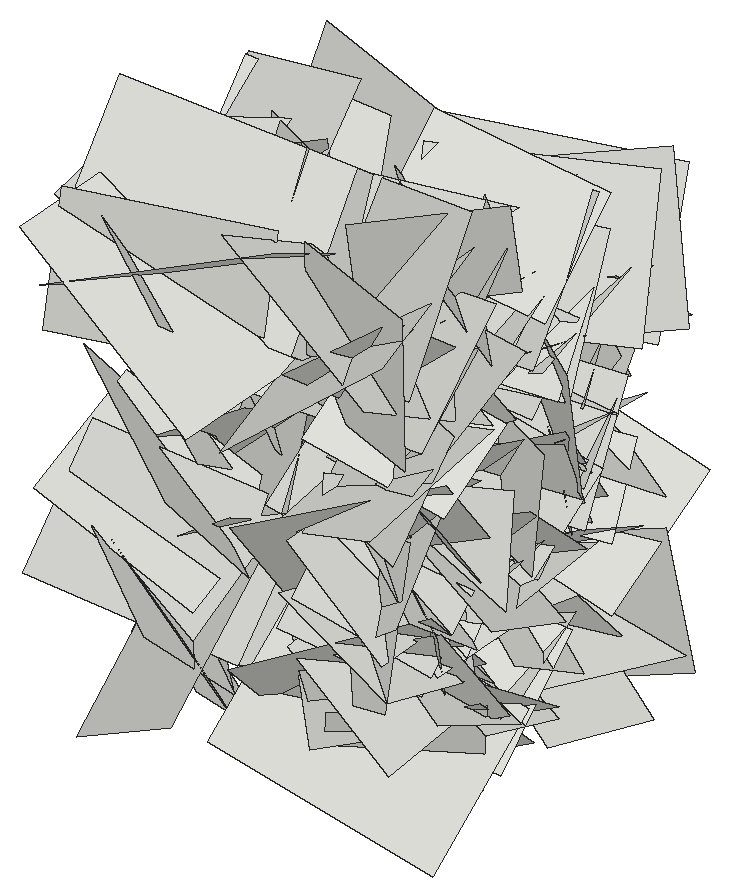
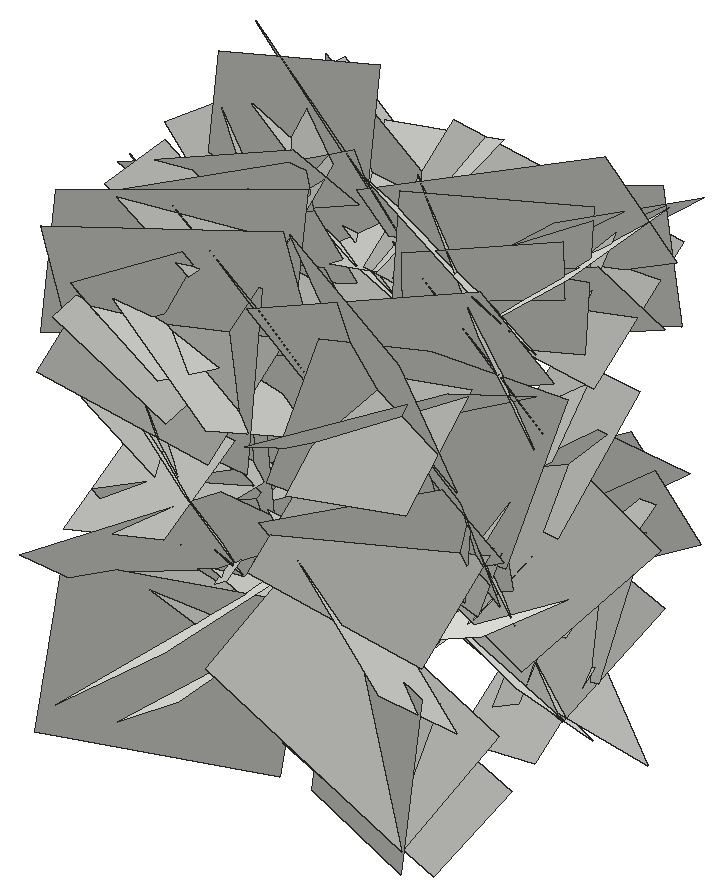
# SketchUp Ruby script. Lengths in inches.
U = 1.inch
M = Sketchup.active_model
def pt(a) = Geom::Point3d.new(a.map { |v| v * U })
def face(e, loops, mat)
  f = e.add_face(loops[0].map { |a| pt(a) })
  loops[1..].each { |l| e.add_face(l.map { |a| pt(a) }).erase! }
  f.material = f.back_material = mat if mat
  f
end
# faces: each face lists its corners as indices into pts; further lists are holes
def faces(e, pts, list, mat = nil) = list.each { |f| face(e, (f[0].is_a?(Array) ? f : [f]).map { |l| l.map { |i| pts[i] } }, mat) }
# xy, xz, yz: faces in a plane at the given z, y or x. An outline is a flat list of corners, or four numbers for a rectangle; further outlines are holes
def ring(l) = l.size == 4 ? [[l[0], l[1]], [l[2], l[1]], [l[2], l[3]], [l[0], l[3]]] : l.each_slice(2).to_a
def flat(e, list, mat, &to3) = list.each { |f| face(e, (f[0].is_a?(Array) ? f : [f]).map { |l| ring(l).map { |u, v| to3.(u, v) } }, mat) }
def xy(e, z, list, mat = nil) = flat(e, list, mat) { |x, y| [x, y, z] }
def xz(e, y, list, mat = nil) = flat(e, list, mat) { |x, z| [x, y, z] }
def yz(e, x, list, mat = nil) = flat(e, list, mat) { |y, z| [x, y, z] }
def lines(e, pts, list) = list.each { |a, b| e.add_line(pt(pts[a]), pt(pts[b])) }
# prism: a flat outline (further loops are holes) pulled along v
def prism(e, loops, v, mat = nil)
  f = face(e, loops, mat); d = Geom::Vector3d.new(v.map { |x| x * U })
  f.pushpull(f.normal.samedirection?(d) ? d.length : -d.length)
end
def box(e, o, s, mat = nil) = prism(e, [[o, [o[0] + s[0], o[1], o[2]], [o[0] + s[0], o[1] + s[1], o[2]], [o[0], o[1] + s[1], o[2]]]], [0, 0, s[2]], mat)
def at(x, y, z, deg = 0) = Geom::Transformation.translation(pt([x, y, z])) * Geom::Transformation.rotation(ORIGIN, Z_AXIS, deg.degrees)
def axes(o, x, y, z) = Geom::Transformation.new([*x, 0, *y, 0, *z, 0, *pt(o).to_a, 1])
def part(name) = M.definitions.add(name)
# library, detail: a bought-in or finely detailed component or shape, given as its bounding box
def library(name, o, s) = part(name).tap { |d| box(d.entities, o, s) }
def detail(e, o, s) = box(e.add_group.entities, o, s)
def put(e, d, t, mat = nil) = e.add_instance(d, t).tap { |i| i.material = mat if mat }
def group(e, t, mat = nil) = e.add_group.tap { |g| g.transformation = t; g.material = mat if mat }.entities
root = M.entities
c1 = part("Component\#6")
p = [[0.01,0,0],[0,3.24,4.54],[4.32,3.24,4.54],[4.33,0,0]]
faces(c1.entities,p,[[0,1,2,3]])
put(root,c1,axes([18.5,168.24,29.62],[0.00844,-0.1319,-0.59476],[0.00779,-0.59475,0.132],[-0.64572,-0.0089,-0.00618]))
put(root,c1,axes([14.53,168.37,37.02],[-0.06582,-0.55881,-0.84289],[0.17414,-0.83883,0.54402],[1.05774,0.10333,-0.14201]))
put(root,c1,axes([14.53,162.55,24.47],[0.08094,0.6993,-0.63815],[0.06519,-0.64254,-0.69674],[1.00139,-0.01469,0.09694]))
put(root,c1,axes([18.5,167.47,38.84],[0.19203,-0.25676,-0.78485],[0.09527,-0.79261,0.28005],[-0.87013,-0.14344,-0.14255]))
put(root,c1,axes([18.5,168.14,25.37],[0.00005,-0.54267,0.44601],[0.16088,0.43548,0.52984],[-0.72699,0.09633,0.11728]))
put(root,c1,axes([14.53,169.13,31.47],[0.22896,-0.22184,-0.76377],[0.12794,-0.77313,0.25869],[0.83329,0.17965,0.17014]))
put(root,c1,axes([14.53,164.67,22.86],[-0.07455,-1.03669,0.46758],[0.01691,0.46753,1.03897],[1.20537,-0.07068,0.01434]))
put(root,c1,axes([18.5,161.42,33.85],[0.12931,-0.58697,0.4315],[0.06321,0.44408,0.58723],[-0.76963,-0.06214,0.12073]))
put(root,c1,axes([14.53,160.7,27.63],[-0.09928,0.64406,-0.88513],[0.13228,-0.87629,-0.65083],[1.15276,0.15602,-0.00154]))
put(root,c1,axes([14.53,159.57,38.3125],[-0.19748,1.37219,0.09956],[-0.15298,0.08042,-1.37849],[1.4503,0.19533,-0.13185]))
put(root,c1,axes([18.5,165.91,24.52],[-0.03596,-0.58924,0.24858],[0.15481,0.23521,0.57749],[-0.65999,0.08727,0.12191]))
put(root,c1,axes([14.53,166.55,31.56],[0.0814,0.41102,-0.8284],[0.17089,-0.82447,-0.39413],[0.96524,0.11131,0.13964]))
put(root,c1,axes([18.5,169.1,21.1],[0.05323,-0.42134,0.48328],[0.06346,0.48572,0.41725],[-0.67666,0.01241,0.07715]))
put(root,c1,axes([14.53,166.67,25.47],[-0.29316,-1.18227,0.54308],[0.10516,0.53443,1.21398],[1.37509,-0.29293,0.02294]))
put(root,c1,axes([14.53,168.75,37.98],[-0.06882,-0.53698,-1.12739],[-0.1022,-1.12338,0.54063],[1.31971,-0.115,-0.01692]))
put(root,c1,axes([14.53,158.58,28.72],[0.17742,0.80309,0.64454],[-0.10421,0.66248,-0.79991],[1.08655,-0.0676,-0.18196]))
put(root,c1,axes([18.5,163.1,21.29],[0.03251,-0.459,0.52355],[0.17075,0.51451,0.44164],[-0.71801,0.10157,0.12873]))
put(root,c1,axes([14.53,169.04,36.23],[-0.04162,0.78981,-0.64322],[0.24351,-0.62024,-0.77563],[1.05189,0.17484,0.15411]))
put(root,c1,axes([14.53,170.89,20.28],[0.12274,-1.02279,0.17958],[-0.0333,0.17716,1.02926],[1.10024,0.11946,0.01112]))
put(root,c1,axes([14.53,167.53,29.6],[0.04916,0.6172,0.8297],[0.08211,0.82613,-0.61887],[1.09305,-0.08981,0.00917]))
put(root,c1,axes([14.53,171.44,27.64],[0.05126,-0.8571,0.56567],[0.11133,0.56746,0.85083],[1.08285,-0.01777,-0.11425]))
put(root,c1,axes([18.5,163.13,28.77],[0.13219,-0.55975,0.33448],[0.05965,0.34851,0.56225],[-0.68862,-0.07726,0.11291]))
put(root,c1,axes([14.53,163.625,35.04],[0.27654,-0.44632,0.88094],[-0.09901,0.89592,0.48157],[1.04211,0.20356,-0.18801]))
put(root,c1,axes([14.53,167.41,29.34],[-0.20833,-0.42173,1.22713],[0.0869,1.23461,0.43743],[1.37269,-0.14217,0.15855]))
put(root,c1,axes([14.53,168.84,39.14],[0.0295,-0.69575,-0.73723],[0.22295,-0.71749,0.68506],[1.05113,0.17171,-0.12461]))
put(root,c1,axes([14.53,163.85,26.9],[0.03329,1.04875,0.11229],[0.24045,0.10299,-1.02538],[1.09187,-0.05466,0.22238]))
put(root,c1,axes([14.53,160.22,28.4],[0.15479,0.80897,-0.76348],[-0.02106,-0.76802,-0.81757],[1.17891,-0.11994,0.08565]))
put(root,c1,axes([14.53,169.63,32.59],[0.01533,-0.4611,-1.03377],[0.17767,-1.02158,0.45801],[1.18663,0.15892,-0.05522]))
put(root,c1,axes([14.53,159.8,34.2],[-0.03301,0.77795,0.85676],[0.24326,0.8442,-0.75821],[1.20233,-0.14944,0.17692]))
put(root,c1,axes([14.53,166.97,25.06],[-0.03339,-0.82276,-0.77538],[0.30966,-0.75526,0.78954],[1.15769,0.17829,-0.23355]))
put(root,c1,axes([14.53,165.55,34.43],[-0.04885,1.13911,0.54464],[0.08516,0.54654,-1.13629],[1.33566,0.00681,0.09237]))
put(root,c1,axes([14.53,164.92,23.28],[0.02573,-1.02703,-0.88101],[-0.12942,-0.87922,1.02158],[1.42847,-0.06116,0.10843]))
put(root,c1,axes([14.53,160.96,32.62],[0.12215,0.75895,-0.88724],[0.014,-0.89234,-0.7616],[1.23753,-0.06482,0.09619]))
put(root,c1,axes([14.53,172.54,38.57],[-0.12011,-0.4932,-1.18141],[0.20578,-1.17893,0.47355],[1.34134,0.1367,-0.17844]))
put(root,c1,axes([14.53,171.44,26.6],[-0.03428,0.27698,-1.26013],[0.06702,-1.25867,-0.27828],[1.36598,0.0687,-0.01797]))
put(root,c1,axes([14.53,173.53,27.66],[0.08068,-0.97468,-0.75893],[0.01331,-0.75972,0.97695],[1.30935,0.06778,0.03684]))
put(root,c1,axes([14.53,158.99,33.95],[0.09747,0.08794,1.12692],[0.17247,1.11783,-0.1005],[1.18568,-0.16983,-0.07802]))
put(root,c1,axes([14.53,166.62,31.96],[0.21061,0.75098,-0.921],[-0.02022,-0.93165,-0.76377],[1.25951,-0.14053,0.14175]))
put(root,c1,axes([14.53,158.06,26.05],[0.19995,0.52409,1.06255],[0.00833,1.07535,-0.5318],[1.25583,-0.09057,-0.16565]))
put(root,c1,axes([14.53,172.42,21.79],[0.22827,-1.35966,0.24048],[-0.1567,0.21929,1.3722],[1.45519,0.2369,0.11004]))
put(root,c1,axes([14.53,165.11,34.6875],[0.03998,0.77126,1.05992],[0.2457,1.03973,-0.76482],[1.36759,-0.20934,0.10642]))
put(root,c1,axes([14.53,159.18,36.25],[0.04304,0.74935,1.15311],[0.14712,1.14549,-0.74928],[1.45028,-0.13844,0.04179]))
put(root,c1,axes([14.53,168.45,29.92],[0.2904,-0.81126,-1.09363],[-0.15157,-1.12651,0.79984],[1.4354,0.04517,0.30571]))
put(root,c1,axes([14.53,157.9,37.93],[0.24747,1.3445,0.30187],[-0.11522,0.32319,-1.35538],[1.4561,-0.20293,-0.15855]))
put(root,c1,axes([14.53,163.2,33.68],[0.16473,-1.2102,0.57798],[0.2383,0.59712,1.18983],[1.40149,0.04071,-0.27024]))
put(root,c1,axes([28.31,163.2,33.68],[-0.16473,-1.2102,0.57798],[-0.2383,0.59712,1.18983],[-1.40149,0.04071,-0.27024]))
put(root,c1,axes([28.31,157.9,37.93],[-0.24747,1.3445,0.30187],[0.11522,0.32319,-1.35538],[-1.4561,-0.20293,-0.15855]))
put(root,c1,axes([28.31,168.45,29.92],[-0.2904,-0.81126,-1.09363],[0.15157,-1.12651,0.79984],[-1.4354,0.04517,0.30571]))
put(root,c1,axes([28.31,159.18,36.25],[-0.04304,0.74935,1.15311],[-0.14712,1.14549,-0.74928],[-1.45028,-0.13844,0.04179]))
put(root,c1,axes([28.31,165.11,34.6875],[-0.03998,0.77126,1.05992],[-0.2457,1.03973,-0.76482],[-1.36759,-0.20934,0.10642]))
put(root,c1,axes([28.31,172.42,21.79],[-0.22827,-1.35966,0.24048],[0.1567,0.21929,1.3722],[-1.45519,0.2369,0.11004]))
put(root,c1,axes([28.31,158.06,26.05],[-0.19995,0.52409,1.06255],[-0.00833,1.07535,-0.5318],[-1.25583,-0.09057,-0.16565]))
put(root,c1,axes([28.31,166.62,31.96],[-0.21061,0.75098,-0.921],[0.02022,-0.93165,-0.76377],[-1.25951,-0.14053,0.14175]))
put(root,c1,axes([28.31,158.99,33.95],[-0.09747,0.08794,1.12692],[-0.17247,1.11783,-0.1005],[-1.18568,-0.16983,-0.07802]))
put(root,c1,axes([28.31,173.53,27.66],[-0.08068,-0.97468,-0.75893],[-0.01331,-0.75972,0.97695],[-1.30935,0.06778,0.03684]))
put(root,c1,axes([28.31,171.44,26.6],[0.03428,0.27698,-1.26013],[-0.06702,-1.25867,-0.27828],[-1.36598,0.0687,-0.01797]))
put(root,c1,axes([28.31,172.54,38.57],[0.12011,-0.4932,-1.18141],[-0.20578,-1.17893,0.47355],[-1.34134,0.1367,-0.17844]))
put(root,c1,axes([28.31,160.96,32.62],[-0.12215,0.75895,-0.88724],[-0.014,-0.89234,-0.7616],[-1.23753,-0.06482,0.09619]))
put(root,c1,axes([28.31,164.92,23.28],[-0.02573,-1.02703,-0.88101],[0.12942,-0.87922,1.02158],[-1.42847,-0.06116,0.10843]))
put(root,c1,axes([28.31,165.55,34.43],[0.04885,1.13911,0.54464],[-0.08516,0.54654,-1.13629],[-1.33566,0.00681,0.09237]))
put(root,c1,axes([28.31,166.97,25.06],[0.03339,-0.82276,-0.77538],[-0.30966,-0.75526,0.78954],[-1.15769,0.17829,-0.23355]))
put(root,c1,axes([28.31,159.8,34.2],[0.03301,0.77795,0.85676],[-0.24326,0.8442,-0.75821],[-1.20233,-0.14944,0.17692]))
put(root,c1,axes([28.31,169.63,32.59],[-0.01533,-0.4611,-1.03377],[-0.17767,-1.02158,0.45801],[-1.18663,0.15892,-0.05522]))
put(root,c1,axes([28.31,160.22,28.4],[-0.15479,0.80897,-0.76348],[0.02106,-0.76802,-0.81757],[-1.17891,-0.11994,0.08565]))
put(root,c1,axes([28.31,163.85,26.9],[-0.03329,1.04875,0.11229],[-0.24045,0.10299,-1.02538],[-1.09187,-0.05466,0.22238]))
put(root,c1,axes([28.31,168.84,39.14],[-0.0295,-0.69575,-0.73723],[-0.22295,-0.71749,0.68506],[-1.05113,0.17171,-0.12461]))
put(root,c1,axes([28.31,167.41,29.34],[0.20833,-0.42173,1.22713],[-0.0869,1.23461,0.43743],[-1.37269,-0.14217,0.15855]))
put(root,c1,axes([28.31,163.625,35.04],[-0.27654,-0.44632,0.88094],[0.09901,0.89592,0.48157],[-1.04211,0.20356,-0.18801]))
put(root,c1,axes([24.34,163.13,28.77],[-0.13219,-0.55975,0.33448],[-0.05965,0.34851,0.56225],[0.68862,-0.07726,0.11291]))
put(root,c1,axes([28.31,171.44,27.64],[-0.05126,-0.8571,0.56567],[-0.11133,0.56746,0.85083],[-1.08285,-0.01777,-0.11425]))
put(root,c1,axes([28.31,167.53,29.6],[-0.04916,0.6172,0.8297],[-0.08211,0.82613,-0.61887],[-1.09305,-0.08981,0.00917]))
put(root,c1,axes([28.31,170.89,20.28],[-0.12274,-1.02279,0.17958],[0.0333,0.17716,1.02926],[-1.10024,0.11946,0.01112]))
put(root,c1,axes([28.31,169.04,36.23],[0.04162,0.78981,-0.64322],[-0.24351,-0.62024,-0.77563],[-1.05189,0.17484,0.15411]))
put(root,c1,axes([24.34,163.1,21.29],[-0.03251,-0.459,0.52355],[-0.17075,0.51451,0.44164],[0.71801,0.10157,0.12873]))
put(root,c1,axes([28.31,158.58,28.72],[-0.17742,0.80309,0.64454],[0.10421,0.66248,-0.79991],[-1.08655,-0.0676,-0.18196]))
put(root,c1,axes([28.31,168.75,37.98],[0.06882,-0.53698,-1.12739],[0.1022,-1.12338,0.54063],[-1.31971,-0.115,-0.01692]))
put(root,c1,axes([28.31,166.67,25.47],[0.29316,-1.18227,0.54308],[-0.10516,0.53443,1.21398],[-1.37509,-0.29293,0.02294]))
put(root,c1,axes([24.34,169.1,21.1],[-0.05323,-0.42134,0.48328],[-0.06346,0.48572,0.41725],[0.67666,0.01241,0.07715]))
put(root,c1,axes([28.31,166.55,31.56],[-0.0814,0.41102,-0.8284],[-0.17089,-0.82447,-0.39413],[-0.96524,0.11131,0.13964]))
put(root,c1,axes([24.34,165.91,24.52],[0.03596,-0.58924,0.24858],[-0.15481,0.23521,0.57749],[0.65999,0.08727,0.12191]))
put(root,c1,axes([28.31,159.57,38.3125],[0.19748,1.37219,0.09956],[0.15298,0.08042,-1.37849],[-1.4503,0.19533,-0.13185]))
put(root,c1,axes([28.31,160.7,27.63],[0.09928,0.64406,-0.88513],[-0.13228,-0.87629,-0.65083],[-1.15276,0.15602,-0.00154]))
put(root,c1,axes([24.34,161.42,33.85],[-0.12931,-0.58697,0.4315],[-0.06321,0.44408,0.58723],[0.76963,-0.06214,0.12073]))
put(root,c1,axes([28.31,164.67,22.86],[0.07455,-1.03669,0.46758],[-0.01691,0.46753,1.03897],[-1.20537,-0.07068,0.01434]))
put(root,c1,axes([28.31,169.13,31.47],[-0.22896,-0.22184,-0.76377],[-0.12794,-0.77313,0.25869],[-0.83329,0.17965,0.17014]))
put(root,c1,axes([24.34,168.14,25.37],[-0.00005,-0.54267,0.44601],[-0.16088,0.43548,0.52984],[0.72699,0.09633,0.11728]))
put(root,c1,axes([24.34,167.47,38.84],[-0.19203,-0.25676,-0.78485],[-0.09527,-0.79261,0.28005],[0.87013,-0.14344,-0.14255]))
put(root,c1,axes([28.31,162.55,24.47],[-0.08094,0.6993,-0.63815],[-0.06519,-0.64254,-0.69674],[-1.00139,-0.01469,0.09694]))
put(root,c1,axes([28.31,168.37,37.02],[0.06582,-0.55881,-0.84289],[-0.17414,-0.83883,0.54402],[-1.05774,0.10333,-0.14201]))
put(root,c1,axes([24.34,168.24,29.62],[-0.00844,-0.1319,-0.59476],[-0.00779,-0.59475,0.132],[0.64572,-0.0089,-0.00618]))
put(root,c1,axes([24.34,163.79,31.02],[-0.0186,-0.39942,0.51021],[-0.04828,0.50989,0.39761],[0.68514,0.02509,0.04187]))
put(root,c1,axes([24.34,167.3,30.05],[-0.09755,-0.36279,0.79394],[-0.2327,0.7823,0.33203],[0.89554,0.16375,0.17276]))
put(root,c1,axes([24.34,166.74,28.03],[-0.20581,0.5378,0.53941],[0.0447,0.5634,-0.54654],[0.80617,0.10606,0.16802]))
put(root,c1,axes([24.34,165.16,26.22],[0.00662,-0.41647,0.48084],[-0.04981,0.47925,0.41571],[0.67246,0.0396,0.02606]))
put(root,c1,axes([28.31,162.15,25.43],[0.09766,0.84172,-0.54191],[-0.18116,-0.52299,-0.84139],[-1.04557,0.16923,0.09516]))
put(root,c1,axes([24.34,170.38,37.22],[-0.01844,-0.65259,0.06973],[-0.0154,0.07012,0.65262],[0.69551,-0.01575,0.0163]))
put(root,c1,axes([28.31,159.15,32.85],[0.28722,0.93511,0.86971],[0.00467,0.88838,-0.95656],[-1.35365,0.20148,0.18123]))
put(root,c1,axes([24.34,158.35,30.49],[-0.08461,0.81055,-0.03501],[-0.12527,-0.04642,-0.80528],[0.85081,0.07377,-0.12204]))
put(root,c1,axes([24.34,168.23,31.98],[-0.11552,-0.73847,0.10601],[0.00435,0.10653,0.74638],[0.79079,-0.10846,0.01138]))
put(root,c1,axes([24.34,162.33,29.83],[-0.22776,0.38392,-0.75072],[0.01782,-0.77261,-0.39993],[0.89361,0.11326,-0.18337]))
put(root,c1,axes([28.31,165.04,27.71],[0.04822,0.07219,0.94774],[-0.14201,0.93984,-0.06516],[-0.99746,-0.13032,0.05509]))
put(root,c1,axes([24.34,171.91,32.4],[0.07209,-0.36069,-0.54144],[-0.07785,-0.54516,0.35394],[0.6852,-0.024,0.09718]))
put(root,c1,axes([28.31,167.29,35.58],[-0.17595,-0.29467,-0.74084],[-0.05215,-0.7515,0.30993],[-0.84352,0.10793,0.13537]))
put(root,c1,axes([28.31,157.3125,32.29],[0.25179,1.05256,0.51222],[-0.06429,0.53303,-1.06718],[-1.23914,0.18623,0.15945]))
put(root,c1,axes([24.34,168.82,35.84],[0.04533,0.37689,0.51175],[-0.01637,0.51337,-0.3768],[0.67349,-0.01289,-0.04361]))
put(root,c1,axes([24.34,159.46,22.85],[-0.09982,-0.0635,0.89488],[-0.1784,0.88507,0.04509],[0.93408,0.16225,0.10424]))
put(root,c1,axes([24.34,160.06,22.6],[-0.02839,-0.24478,0.77995],[-0.15528,0.76918,0.23637],[0.85248,0.13195,0.06903]))
put(root,c1,axes([24.34,159.67,28.14],[-0.12868,0.67272,0.52517],[-0.08613,0.51893,-0.68352],[0.90053,0.14576,0.00967]))
put(root,c1,axes([24.34,158.39,26.84],[-0.02686,0.84806,0.10272],[-0.17857,0.09579,-0.83237],[0.88773,0.04493,-0.16432]))
put(root,c1,axes([24.34,169.17,27.35],[0.00515,-0.4485,-0.48712],[0.04455,-0.48594,0.44784],[0.70046,0.0342,-0.02491]))
put(root,c1,axes([28.31,161.79,25.53],[-0.01152,-0.82607,0.19056],[-0.15176,0.18963,0.81386],[-0.88572,-0.02175,-0.14193]))
put(root,c1,axes([28.31,164.2,31.01],[0.06613,-0.18181,-0.96198],[-0.02897,-0.96387,0.1804],[-1.03734,0.01533,-0.06637]))
put(root,c1,axes([24.34,169.92,30.86],[0.08798,0.07784,-0.70174],[-0.08853,-0.70052,-0.08758],[0.74315,-0.09267,0.07264]))
put(root,c1,axes([28.31,162.32,28.44],[-0.12821,-0.42216,-0.69512],[0.01339,-0.70366,0.42514],[-0.86197,0.05186,0.11]))
put(root,c1,axes([28.31,166.33,22.3],[0.05809,-0.87115,0.26873],[-0.09257,0.26296,0.87026],[-0.96191,-0.07791,-0.06752]))
put(root,c1,axes([28.31,171.77,39.47],[0.25632,-0.1505,-1.28885],[0.2021,-1.29268,0.18672],[-1.36053,-0.22038,-0.21508]))
put(root,c1,axes([24.34,167.69,34.89],[0.01272,-0.59445,-0.3878],[0.01652,-0.38754,0.59453],[0.75216,0.01856,-0.0065]))
put(root,c1,axes([24.34,168.18,25.35],[0.0356,-0.79141,-0.13903],[-0.13499,-0.14264,0.78117],[0.84098,0.01061,0.13127]))
put(root,c1,axes([28.31,163.85,33.45],[0.03445,-0.73428,-0.4148],[-0.17499,-0.41262,0.71747],[-0.87664,0.05351,-0.15952]))
put(root,c1,axes([28.31,158.45,30.92],[0.16236,0.46297,0.88251],[-0.09478,0.89566,-0.45434],[-1.05211,-0.00924,0.17712]))
put(root,c1,axes([28.31,166.53,31.68],[0.02185,0.89564,-0.0065],[-0.05171,-0.00537,-0.89456],[-0.948,0.02094,0.04865]))
put(root,c1,axes([28.31,171.21,38.93],[0.24063,-0.51313,-1.11059],[0.16085,-1.10901,0.54342],[-1.28679,-0.23458,-0.13976]))
put(root,c1,axes([24.34,171.89,34.33],[-0.10287,-0.74562,-0.1631],[0.15609,-0.17961,0.73351],[0.79385,-0.06131,-0.16536]))
put(root,c1,axes([28.31,162.43,26.35],[-0.02315,-0.70596,0.51236],[0.01203,0.51225,0.70629],[-0.92456,0.02434,-0.00364]))
put(root,c1,axes([28.31,162.61,28.57],[0.04222,-0.49534,0.62953],[-0.20196,0.60636,0.48917],[-0.82474,-0.17384,-0.08755]))
put(root,c1,axes([28.31,162.92,24.26],[-0.16568,0.16434,-0.80239],[0.1251,-0.80382,-0.18763],[-0.85913,-0.14874,0.12742]))
put(root,c1,axes([28.31,164.5,23.79],[-0.04443,0.667,0.37408],[-0.11412,0.36576,-0.66423],[-0.80255,-0.08894,0.07374]))
put(root,c1,axes([28.31,168.875,35.8],[-0.07444,0.7996,-0.0855],[-0.00091,-0.0859,-0.80263],[-0.85241,-0.06974,0.00832]))
put(root,c1,axes([24.34,164.96,33.58],[0.03363,-0.67551,-0.53197],[-0.14584,-0.52946,0.66412],[0.89967,-0.06058,0.12754]))
put(root,c1,axes([24.34,169.82,24.93],[0.00586,-0.68753,0.27068],[0.05817,0.27032,0.6855],[0.78107,-0.01497,-0.05308]))
put(root,c1,axes([28.31,164.8,26.41],[-0.06555,-0.88967,-0.10275],[0.1194,-0.1099,0.88381],[-0.94178,0.04799,0.1192]))
put(root,c1,axes([28.31,163.99,40.83],[-0.08038,0.23372,-0.81219],[0.10222,-0.80774,-0.24144],[-0.89001,-0.11388,0.04562]))
put(root,c1,axes([28.31,167.51,23.32],[0.04127,-0.8056,0.43064],[0.05085,0.43224,0.80425],[-0.96695,-0.01165,0.06068]))
put(root,c1,axes([28.31,164.95,29.96],[0.04265,0.57286,-0.52342],[-0.15347,-0.50938,-0.56862],[-0.80809,0.12697,0.08036]))
